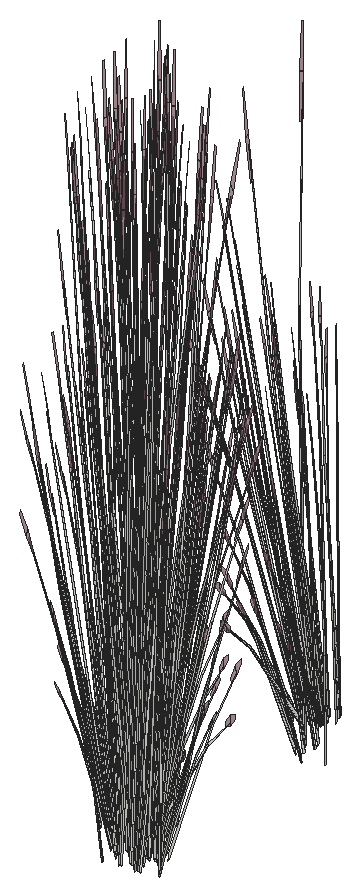
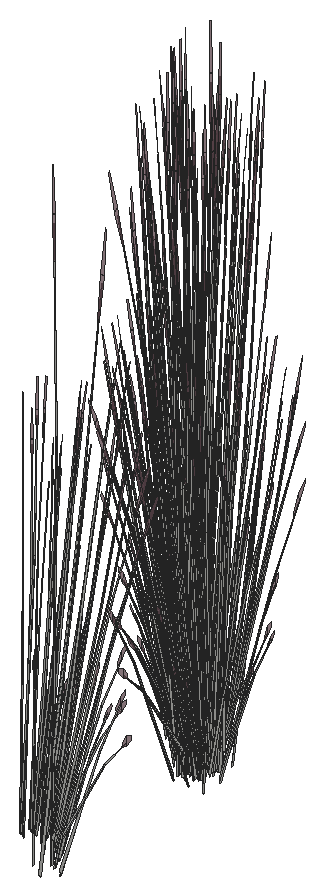
# SketchUp Ruby script. Lengths in inches.
U = 1.inch
M = Sketchup.active_model
def pt(a) = Geom::Point3d.new(a.map { |v| v * U })
def face(e, loops, mat)
  f = e.add_face(loops[0].map { |a| pt(a) })
  loops[1..].each { |l| e.add_face(l.map { |a| pt(a) }).erase! }
  f.material = f.back_material = mat if mat
  f
end
# faces: each face lists its corners as indices into pts; further lists are holes
def faces(e, pts, list, mat = nil) = list.each { |f| face(e, (f[0].is_a?(Array) ? f : [f]).map { |l| l.map { |i| pts[i] } }, mat) }
# xy, xz, yz: faces in a plane at the given z, y or x. An outline is a flat list of corners, or four numbers for a rectangle; further outlines are holes
def ring(l) = l.size == 4 ? [[l[0], l[1]], [l[2], l[1]], [l[2], l[3]], [l[0], l[3]]] : l.each_slice(2).to_a
def flat(e, list, mat, &to3) = list.each { |f| face(e, (f[0].is_a?(Array) ? f : [f]).map { |l| ring(l).map { |u, v| to3.(u, v) } }, mat) }
def xy(e, z, list, mat = nil) = flat(e, list, mat) { |x, y| [x, y, z] }
def xz(e, y, list, mat = nil) = flat(e, list, mat) { |x, z| [x, y, z] }
def yz(e, x, list, mat = nil) = flat(e, list, mat) { |y, z| [x, y, z] }
def lines(e, pts, list) = list.each { |a, b| e.add_line(pt(pts[a]), pt(pts[b])) }
# prism: a flat outline (further loops are holes) pulled along v
def prism(e, loops, v, mat = nil)
  f = face(e, loops, mat); d = Geom::Vector3d.new(v.map { |x| x * U })
  f.pushpull(f.normal.samedirection?(d) ? d.length : -d.length)
end
def box(e, o, s, mat = nil) = prism(e, [[o, [o[0] + s[0], o[1], o[2]], [o[0] + s[0], o[1] + s[1], o[2]], [o[0], o[1] + s[1], o[2]]]], [0, 0, s[2]], mat)
def at(x, y, z, deg = 0) = Geom::Transformation.translation(pt([x, y, z])) * Geom::Transformation.rotation(ORIGIN, Z_AXIS, deg.degrees)
def axes(o, x, y, z) = Geom::Transformation.new([*x, 0, *y, 0, *z, 0, *pt(o).to_a, 1])
def part(name) = M.definitions.add(name)
# library, detail: a bought-in or finely detailed component or shape, given as its bounding box
def library(name, o, s) = part(name).tap { |d| box(d.entities, o, s) }
def detail(e, o, s) = box(e.add_group.entities, o, s)
def put(e, d, t, mat = nil) = e.add_instance(d, t).tap { |i| i.material = mat if mat }
def group(e, t, mat = nil) = e.add_group.tap { |g| g.transformation = t; g.material = mat if mat }.entities
root = M.entities
M.materials.add("LightPink_Translucent").color = [144, 107, 117]
M.materials["LightPink_Translucent"].alpha = 0.75
c1 = part("blade")
p = [[2.15,0.21,22],[0,0.17,0],[0.09,0.45,0],[2.18,0.31,22],[2.29,0.31,22],[0.38,0.45,0],
  [2.48,0.24,33],[2.49,0.24,33],[2.48,0.22,33]]
faces(c1.entities,p,[[0,1,2,3],[4,5,2,3],[6,3,4,7],[8,0,3,6]])
c2 = part("seeds")
p = [[0.3,-0.1,1.38],[-0.01,-0.03,1.59],[-0.01,-0.03,0.03],[0.14,-0.07,-0.07],[0.29,-0.03,3],[0.15,0.01,3.11]]
faces(c2.entities,p,[[0,1,2,3],[1,0,4,5]],"LightPink_Translucent")
c3 = part("blade with seeds")
put(c3.entities,c1,at(0,0,0))
put(c3.entities,c2,axes([2.4,0.25,30.99],[1.5799,-0.05474,1.17369],[-0.12525,1.92788,0.29478],[-0.07173,-0.02425,1.56792]))
put(root,c3,axes([332.67,539,1402.53],[0.30722,-0.06665,-0.35414],[0.08112,0.381,0.4572],[0.08804,-0.10234,0.87481]))
put(root,c3,axes([329.78,538.36,1402.73],[0.01777,-0.35463,0.0643],[0.26836,0.00972,0.50621],[-0.1028,-0.03711,0.77189]))
put(root,c3,axes([330.71,539.55,1400.21],[0.17124,-0.42022,-0.44739],[0.35581,0.20224,0.21531],[0,-0.09687,1.43643]))
put(root,c3,axes([329.68,538.47,1402.53],[-0.20082,-0.29199,-0.35414],[0.2293,-0.2764,0.4572],[-0.1165,-0.04206,0.87481]))
put(root,c3,axes([330.86,539.34,1400.67],[-0.04113,-0.53214,-0.29095],[0.42835,-0.03218,-0.50002],[0.07543,-0.07088,1.59708]))
put(root,c3,axes([329.8,539.37,1400.03],[0.24637,-0.29097,-0.30978],[0.24637,0.29097,0.30978],[0,-0.09372,1.38974]))
put(root,c3,axes([329.7,537.97,1400.13],[-0.10181,0.3808,-0.03893],[-0.31336,-0.11714,-0.17649],[-0.04758,-0.06228,0.58215]))
put(root,c3,axes([332.42,539.22,1403.05],[-0.30722,0.06665,0.35414],[-0.08112,-0.381,-0.4572],[0.08804,-0.10234,0.87481]))
put(root,c3,axes([330.67,539.9,1400.67],[-0.39748,-0.22252,-0.29095],[0.19139,-0.46966,-0.50002],[-0.01249,-0.11531,1.59708]))
put(root,c3,axes([329.53,539.71,1400.375],[-0.44133,0,0],[0,-0.52122,-0.51607],[0,-0.11871,1.63711]))
put(root,c3,axes([329.61,538.78,1400.59],[0.06891,0.12984,1.43002],[-0.15879,0.35293,-0.30754],[-0.16304,-0.08436,0.61141]))
put(root,c3,axes([330.81,538.16,1400.03],[0.32928,0.11539,-0.30978],[-0.08291,0.40636,0.30978],[0.06638,-0.04686,1.38974]))
put(root,c3,axes([329.89,538.67,1402.98],[-0.35281,-0.01123,-0.71045],[0.0237,-0.47284,0.08574],[-0.14947,-0.0499,1.00501]))
put(root,c3,axes([332.7,539.16,1402.73],[0.2423,0.19613,0.0643],[-0.14107,0.2793,0.50621],[0.07768,-0.0903,0.77189]))
put(root,c3,axes([332.63,539.08,1402.73],[0.08753,0.42921,0.48003],[-0.34336,0.07449,0.3958],[0.1012,-0.10094,0.9933]))
put(root,c3,axes([333.55,539.6,1402.72],[0.04898,-0.07104,1.74944],[-0.06269,-0.43574,-0.27667],[0.12289,-0.08262,0.14031]))
put(root,c3,axes([329.875,539.58,1400.33],[-0.32829,0.39208,0.30756],[-0.32849,-0.38796,-0.36492],[-0.01146,-0.11134,1.64885]))
put(root,c3,axes([329.42,537.9,1402.71],[0.02617,0.04654,1.77383],[-0.12614,0.41836,-0.16761],[-0.12775,0.00303,0.31391]))
put(root,c3,axes([330.92,539.76,1400.43],[0.39767,0.22603,0.24065],[-0.19139,0.46966,0.50002],[0,-0.10827,1.60543]))
put(root,c3,axes([330.77,540.39,1400.4375],[0.09355,-0.55261,-0.23429],[0.44354,0.09633,0.51271],[-0.0775,-0.07631,1.5644]))
put(root,c3,axes([329.78,538.76,1402.68],[-0.25628,0.30892,-0.51099],[-0.22444,-0.32634,-0.3958],[-0.13021,-0.047,0.97773]))
put(root,c3,axes([329.97,538.625,1403.05],[0.20082,0.29199,0.35414],[-0.2293,0.2764,-0.4572],[-0.1165,-0.04206,0.87481]))
put(root,c3,axes([329.2,539.17,1400.77],[0.22533,-0.03337,1.1486],[-0.14293,0.29403,0.84392],[-0.11135,-0.04411,0.25299]))
put(root,c3,axes([330.79,539.44,1400.72],[-0.38326,0.02879,0.44739],[-0.03466,-0.47788,-0.21531],[0.06861,-0.04843,1.43643]))
put(root,c3,axes([329.91,538.4375,1403.03],[-0.0189,0.47427,-0.1216],[-0.35781,-0.01296,-0.67495],[-0.13781,-0.03295,1.02557]))
put(root,c3,axes([329.8,539.79,1400.48],[0,0.46636,0.49651],[-0.39487,0,0],[0,-0.10622,1.57504]))
put(root,c3,axes([332.59,540.26,1403.03],[-0.17758,-0.42229,-0.1216],[0.31518,-0.20752,-0.67495],[0.13282,-0.05572,1.02557]))
put(root,c3,axes([332.57,539.9,1402.68],[0.09562,-0.42421,-0.51099],[0.32782,0.1454,-0.3958],[0.13199,-0.0389,0.97773]))
put(root,c3,axes([332.06,538.17,1400.375],[0.22066,-0.46731,0],[0.36918,0.26061,-0.51607],[0.08408,0.05936,1.63711]))
put(root,c3,axes([329.46,539.09,1401.875],[0.14639,-0.01056,1.71376],[-0.09712,0.45778,0.13857],[-0.20862,-0.02831,0.73262]))
put(root,c3,axes([330.73,540.17,1400.21],[-0.21202,-0.39143,-0.44739],[0.32115,-0.27564,0.21531],[-0.06861,-0.04843,1.43643]))
put(root,c3,axes([330.78,539.62,1400.36],[0.15345,0.52148,0.45755],[-0.43845,0.18134,0.17955],[0.00536,-0.09582,1.58856]))
put(root,c3,axes([332.92,540.02,1399.98],[-0.22732,0.05597,1.41583],[-0.03618,-0.44548,0.08104],[0.15921,-0.06743,0.80566]))
put(root,c3,axes([333.34,539.62,1400.26],[-0.21881,-0.29821,-0.06488],[0.23965,-0.27324,-0.29416],[0.0679,-0.01924,0.97024]))
put(root,c3,axes([330.7,540.03,1400.72],[-0.17124,0.42022,0.44739],[-0.35581,-0.20224,-0.21531],[0,-0.09687,1.43643]))
put(root,c3,axes([331.33,539.66,1400.21],[0,-0.53961,0],[0.44133,0,0],[0,0,1.79456]))
put(root,c3,axes([331.87,538.41,1400.48],[-0.33032,-0.23318,0.49651],[0.19744,-0.41812,0],[0.07523,0.05311,1.57504]))
put(root,c3,axes([332.51,540.05,1402.98],[0.31014,-0.20596,-0.71045],[0.17284,0.42397,0.08574],[0.14985,-0.04816,1.00501]))
put(root,c3,axes([330.54,540.32,1400.06],[-0.36714,-0.07646,-0.62353],[0.07747,-0.47163,-0.16365],[-0.10956,-0.05715,1.37633]))
put(root,c3,axes([331.12,539.32,1400.36],[-0.29264,0.42323,0.45755],[-0.34767,-0.3736,0.17955],[0.07055,-0.04224,1.58856]))
put(root,c3,axes([331.44,540.08,1400.3],[-0.32829,-0.4014,-0.06131],[0.32849,-0.40164,0],[-0.01146,-0.01402,1.75571]))
put(root,c3,axes([330.61,538.625,1400.47],[-0.10196,0.46348,0.17642],[-0.3731,-0.13116,0.35086],[0.06445,-0.00226,1.60407]))
put(root,c3,axes([332.47,540.13,1403.05],[-0.29332,-0.1301,0.35414],[0.08555,-0.37955,-0.4572],[0.11809,-0.0348,0.87481]))
put(root,c3,axes([329.4,539.4375,1402.73],[0.09971,-0.42522,0.48003],[0.32782,0.1454,0.3958],[-0.12892,0.02555,0.9933]))
put(root,c3,axes([330.46,539,1399.59],[-0.3474,0.18671,1.28929],[-0.11057,-0.53572,0.50096],[0.21332,0.00891,1.46642]))
put(root,c3,axes([331.39,539.14,1400.62],[0.06809,-0.4162,0.1448],[0.33266,0.07225,-0.41347],[0.06054,0.04274,1.26744]))
put(root,c3,axes([329.37,539.33,1402.73],[-0.12963,-0.31798,0.0643],[0.23638,-0.15564,0.50621],[-0.1042,0.03071,0.77189]))
put(root,c3,axes([330.82,540.13,1400.36],[0.44609,0.09826,0.45755],[-0.09078,0.55493,0.17955],[-0.06519,-0.05359,1.58856]))
put(root,c3,axes([333.17,539.72,1399.49],[-0.01845,-0.0708,1.76342],[0.12793,-0.41416,-0.26939],[0.12905,-0.00596,0.30037]))
put(root,c3,axes([329.36,539.65,1399.49],[0.00895,0.0735,1.76342],[-0.18044,0.38382,-0.26939],[-0.12817,-0.01935,0.30037]))
put(root,c3,axes([331.25,539.25,1400.72],[-0.21202,-0.39143,0.44739],[0.32115,-0.27564,-0.21531],[0.06861,0.04843,1.43643]))
put(root,c3,axes([330.15,541.04,1400.03],[-0.08291,-0.40636,-0.30978],[0.32928,-0.11539,0.30978],[-0.06638,-0.04686,1.38974]))
put(root,c3,axes([330.58,541.01,1400.47],[0.37926,-0.12378,0.17642],[0.09365,0.46065,0.35086],[-0.03382,-0.06712,1.60407]))
put(root,c3,axes([331.36,539.27,1400.67],[0.35635,-0.30962,-0.29095],[0.23697,0.43749,-0.50002],[0.08792,0.04443,1.59708]))
put(root,c3,axes([332.78,540.09,1402.53],[0.29332,0.1301,-0.35414],[-0.08555,0.37955,0.4572],[0.11809,-0.0348,0.87481]))
put(root,c3,axes([330.0625,541.21,1400.02],[-0.33032,-0.23318,-0.49651],[0.19744,-0.41812,0],[-0.07523,-0.05311,1.57504]))
put(root,c3,axes([332.26,538.45,1400.02],[0.33032,0.23318,-0.49651],[-0.19744,0.41812,0],[0.07523,0.05311,1.57504]))
put(root,c3,axes([329.33,539.49,1402.53],[-0.29332,-0.1301,-0.35414],[0.08555,-0.37955,0.4572],[-0.11809,0.0348,0.87481]))
put(root,c3,axes([331.63,539.78,1400.21],[0.39487,0,0],[0,0.48281,0],[0,0,1.78407]))
put(root,c3,axes([330.96,540.39,1400.67],[-0.35635,0.30962,-0.29095],[-0.23697,-0.43749,-0.50002],[-0.08792,-0.04443,1.59708]))
put(root,c3,axes([331.74,538.65,1400.47],[-0.37926,0.12378,0.17642],[-0.09365,-0.46065,0.35086],[0.03382,0.06712,1.60407]))
put(root,c3,axes([331.98,539.62,1401.875],[-0.14639,0.01056,1.71376],[0.09712,-0.45778,0.13857],[0.20862,0.02831,0.73262]))
put(root,c3,axes([332.17,538.625,1400.03],[0.08291,0.40636,-0.30978],[-0.32928,0.11539,0.30978],[0.06638,0.04686,1.38974]))
put(root,c3,axes([332.73,540.25,1402.73],[0.12963,0.31798,0.0643],[-0.23638,0.15564,0.50621],[0.1042,-0.03071,0.77189]))
put(root,c3,axes([331.5,539.53,1400.38],[-0.44609,-0.09826,0.49198],[0.09078,-0.55493,0.19306],[0.06519,0.05359,1.70813]))
put(root,c3,axes([332.71,540.14,1402.73],[-0.09971,0.42522,0.48003],[-0.32782,-0.1454,0.3958],[0.12892,-0.02555,0.9933]))
put(root,c3,axes([331.15,540.9,1400.2],[-0.11516,-0.40207,0],[0.32884,-0.1408,0],[0,0,1.54371]))
put(root,c3,axes([330.93,540.52,1400.62],[-0.06809,0.4162,0.1448],[-0.33266,-0.07225,-0.41347],[-0.06054,-0.04274,1.26744]))
put(root,c3,axes([329.64,539.44,1403.05],[0.29332,0.1301,0.35414],[-0.08555,0.37955,-0.4572],[-0.11809,0.0348,0.87481]))
put(root,c3,axes([331.58,540.85,1400.18],[0.37054,-0.15823,-0.19198],[0.1302,0.45581,0.00008],[0.0409,-0.01749,1.73897]))
put(root,c3,axes([331.71,541.04,1400.47],[0.10196,-0.46348,0.17642],[0.3731,0.13116,0.35086],[-0.06445,0.00226,1.60407]))
put(root,c3,axes([331.62,539.99,1400.21],[0.24637,0.30123,0],[-0.24637,0.30123,0],[0,0,1.69266]))
put(root,c3,axes([330.22,539.42,1401.34],[0.10032,-0.06746,1.77064],[0.0346,0.47103,0.13857],[-0.2173,0.0625,0.63284]))
put(root,c3,axes([332.29,539.86,1400.47],[-0.2773,-0.3397,0.17642],[0.27945,-0.32949,0.35086],[-0.03063,0.06937,1.60407]))
put(root,c3,axes([331.78,539.34,1400.06],[0.36714,0.07646,-0.62353],[-0.07747,0.47163,-0.16365],[0.10956,0.05715,1.37633]))
put(root,c3,axes([333.4,540.17,1400.77],[-0.21807,0.07699,1.1486],[0.10265,-0.31819,0.84392],[0.11568,0.02177,0.25299]))
put(root,c3,axes([331.07,541.09,1400.2],[-0.35581,-0.20937,0],[0.17124,-0.43505,0],[0,0,1.62707]))
put(root,c3,axes([331.36,540.53,1400.46],[-0.34464,-0.37536,-0.25192],[0.29,-0.42149,0.5513],[-0.0928,0.04391,1.68216]))
put(root,c3,axes([330.45,541.25,1400.48],[0.33032,0.23318,0.49651],[-0.19744,0.41812,0],[-0.07523,-0.05311,1.57504]))
put(root,c3,axes([331.62,539.64,1400.72],[0.17124,-0.42022,0.44739],[0.35581,0.20224,-0.21531],[0,0.09687,1.43643]))
put(root,c3,axes([333.3,541.51,1402.71],[-0.03191,-0.04083,1.77383],[0.06981,-0.43764,-0.16761],[0.12571,-0.02796,0.31391]))
put(root,c3,axes([329.14,539.74,1402.72],[-0.05763,0.06055,1.74944],[0.0049,0.44239,-0.27667],[-0.13211,0.05753,0.14031]))
put(root,c3,axes([331.55,539.875,1400.29],[0,0.53934,-0.05637],[-0.44133,0,0],[0,0.01695,1.79368]))
put(root,c3,axes([329.53,539.68,1402.68],[-0.09562,0.42421,-0.51099],[-0.32782,-0.1454,-0.3958],[-0.13199,0.0389,0.97773]))
put(root,c3,axes([329.51,539.32,1403.03],[0.17758,0.42229,-0.1216],[-0.31518,0.20752,-0.67495],[-0.13282,0.05572,1.02557]))
put(root,c3,axes([331.58,539.49,1400.21],[0.21202,0.39143,-0.44739],[-0.32115,0.27564,0.21531],[0.06861,0.04843,1.43643]))
put(root,c3,axes([333.02,541.15,1401.93],[-0.06755,-0.39203,-0.03492],[0.31928,-0.09013,-0.15832],[0.06667,0.02485,0.52218]))
put(root,c3,axes([330.26,541.49,1400.375],[-0.22066,0.46731,0],[-0.36918,-0.26061,-0.51607],[-0.08408,-0.05936,1.63711]))
put(root,c3,axes([332.19,541.14,1403.03],[0.0189,-0.47427,-0.1216],[0.35781,0.01296,-0.67495],[0.13781,0.03295,1.02557]))
put(root,c3,axes([332.52,539.87,1400.48],[0,-0.46636,0.49651],[0.39487,0,0],[0,0.10622,1.57504]))
put(root,c3,axes([331.53,540.22,1400.72],[0.38326,-0.02879,0.44739],[0.03466,0.47788,-0.21531],[-0.06861,0.04843,1.43643]))
put(root,c3,axes([331.77,539.73,1400.62],[0.32884,-0.136,0.1448],[0.11516,0.38837,-0.41347],[0,0.08547,1.26744]))
put(root,c3,axes([332.14,540.95,1403.05],[-0.20082,-0.29199,0.35414],[0.2293,-0.2764,-0.4572],[0.1165,0.04206,0.87481]))
put(root,c3,axes([331.1875,540.45,1400.21],[-0.38326,0.02879,-0.44739],[-0.03466,-0.47788,0.21531],[-0.06861,0.04843,1.43643]))
put(root,c3,axes([332.99,540.68,1400.59],[-0.085,-0.1147,1.43002],[0.1106,-0.37943,-0.30754],[0.17198,0.0514,0.61141]))
put(root,c3,axes([331.47,541.09,1400.2],[0.35581,0.20937,0],[-0.17124,0.43505,0],[0,0,1.74954]))
put(root,c3,axes([332.5,540.85,1402.72],[0.07571,-0.00789,1.74944],[0.20767,-0.36231,-0.27667],[0.13467,0.04783,0.14031]))
put(root,c3,axes([331.61,541.56,1400.19],[-0.21791,-0.46895,-0.05142],[0.36918,-0.26061,0.51607],[-0.09097,0.04465,1.6363]))
put(root,c3,axes([331.53,540.42,1400.62],[0.26075,0.2802,0.1448],[-0.2175,0.31612,-0.41347],[-0.06054,0.04274,1.26744]))
put(root,c3,axes([329.47,540.5,1402.73],[-0.08753,-0.42921,0.48003],[0.34336,-0.07449,0.3958],[-0.1012,0.10094,0.9933]))
put(root,c3,axes([329.41,540.41,1402.73],[-0.2423,-0.19613,0.0643],[0.14107,-0.2793,0.50621],[-0.07768,0.0903,0.77189]))
put(root,c3,axes([329.52,539.9,1401.875],[0.12246,-0.09864,1.71376],[0.1031,0.45582,0.13857],[-0.19225,0.10302,0.73262]))
put(root,c3,axes([332.21,540.91,1402.98],[0.35281,0.01123,-0.71045],[-0.0237,0.47284,0.08574],[0.14947,0.0499,1.00501]))
put(root,c3,axes([331.8125,541.29,1400.48],[0.33032,-0.23318,0.49651],[0.19744,0.41812,0],[-0.07523,0.05311,1.57504]))
put(root,c3,axes([331.34,540.92,1400.29],[0.15345,0.53576,-0.06012],[-0.43845,0.18773,0],[0.00536,0.01871,1.72173]))
put(root,c3,axes([331.51,541.5,1400.03],[-0.32928,-0.11539,-0.30978],[0.08291,-0.40636,0.30978],[-0.06638,0.04686,1.38974]))
put(root,c3,axes([329.14,540.67,1400.59],[0.12266,0.03828,1.43002],[0.07906,0.39104,-0.30754],[-0.16661,0.0732,0.61141]))
put(root,c3,axes([329.6875,540.35,1403.05],[0.30722,-0.06665,0.35414],[0.08112,0.381,-0.4572],[-0.08804,0.10234,0.87481]))
put(root,c3,axes([332.78,539.95,1400.375],[0.44133,0,0],[0,0.52122,-0.51607],[0,0.11871,1.63711]))
put(root,c3,axes([328.5,540.18,1402.71],[0.04504,0.01251,1.77383],[0.13934,0.41205,-0.16761],[-0.0922,0.10815,0.31391]))
put(root,c3,axes([332.61,540.22,1400.2],[-0.44111,-0.00373,-0.04976],[0,-0.52122,0.49943],[-0.01386,0.11865,1.58352]))
put(root,c3,axes([331.65,539.76,1400.67],[0.39748,0.22252,-0.29095],[-0.19139,0.46966,-0.50002],[0.01249,0.11531,1.59708]))
put(root,c3,axes([328.88,541.49,1400.77],[0.14709,-0.21136,1.1486],[0.05804,0.3346,0.84392],[-0.1063,0.05991,0.25299]))
put(root,c3,axes([332.42,541.1,1402.53],[0.20082,0.29199,-0.35414],[-0.2293,0.2764,0.4572],[0.1165,0.04206,0.87481]))
put(root,c3,axes([332.52,540.29,1400.03],[-0.24637,0.29097,-0.30978],[-0.24637,-0.29097,0.30978],[0,0.09372,1.38974]))
put(root,c3,axes([331.46,540.32,1400.67],[0.04113,0.53214,-0.29095],[-0.42835,0.03218,-0.50002],[-0.07543,0.07088,1.59708]))
put(root,c3,axes([332.32,541.22,1402.73],[-0.01777,0.35463,0.0643],[-0.26836,-0.00972,0.50621],[0.1028,0.03711,0.77189]))
put(root,c3,axes([331.61,540.11,1400.21],[-0.17124,0.42022,-0.44739],[-0.35581,-0.20224,0.21531],[0,0.09687,1.43643]))
put(root,c3,axes([329.43,540.58,1402.53],[-0.30722,0.06665,-0.35414],[-0.08112,-0.381,0.4572],[-0.08804,0.10234,0.87481]))
put(root,c3,axes([332.34,541.1,1402.73],[-0.26024,0.30729,0.48003],[-0.22444,-0.32634,0.3958],[0.1221,0.05668,0.9933]))
put(root,c3,axes([328.99,541.4375,1403.65],[0.31145,0.12449,-0.06488],[-0.0958,0.38314,-0.29416],[-0.05094,0.05817,0.97024]))
put(root,c3,axes([331.2,540.73,1400.06],[-0.23773,0.35053,-0.62353],[-0.29532,-0.31785,-0.16365],[-0.09526,0.08744,1.37633]))
put(root,c3,axes([331.52,541.46,1403.05],[-0.05451,-0.37564,0.35414],[0.31161,-0.09919,-0.4572],[0.0837,0.10765,0.87481]))
put(root,c3,axes([331.62,541.32,1400.33],[0.44186,0.15158,0.30756],[-0.11054,0.54181,-0.36492],[-0.07313,0.06781,1.64885]))
put(root,c3,axes([331.59,541.68,1400.02],[-0.33032,0.23318,-0.49651],[-0.19744,-0.41812,0],[-0.07523,0.05311,1.57504]))
put(root,c3,axes([332.6875,540.3,1400.02],[0,0.46636,-0.49651],[-0.39487,0,0],[0,0.10622,1.57504]))
put(root,c3,axes([331.7,540.35,1401.875],[-0.1311,-0.08035,1.71376],[0.27131,-0.33708,0.13857],[0.16909,0.15206,0.73262]))
put(root,c3,axes([331.72,539.3,1402.47],[-0.30498,-0.24231,1.38283],[0.32203,-0.37727,0.59665],[0.0984,0.22736,1.33663]))
put(root,c3,axes([329.53,540.32,1403.03],[0.32648,0.25715,-0.1216],[-0.18809,0.3724,-0.67495],[-0.09224,0.12945,1.02557]))
put(root,c3,axes([332.18,541.27,1400.77],[-0.19872,-0.13409,1.1486],[0.2566,-0.13625,0.84392],[0.06921,0.11541,0.25299]))
put(root,c3,axes([331.49,541.65,1403.03],[0.21031,-0.39918,-0.1216],[0.30457,0.22997,-0.67495],[0.10587,0.11278,1.02557]))
put(root,c3,axes([329.97,540.2,1401.875],[0.08815,-0.14329,1.71376],[0.22258,0.38678,0.13857],[-0.15267,0.17614,0.73262]))
put(root,c3,axes([329.6875,540.625,1402.68],[0.09067,0.42583,-0.51099],[-0.34336,0.07449,-0.3958],[-0.0984,0.11438,0.97773]))
put(root,c3,axes([330.1,541.11,1403.05],[0.23881,-0.24554,0.35414],[0.22606,0.28036,-0.4572],[-0.0344,0.14245,0.87481]))
put(root,c3,axes([331.89,541.61,1400.375],[0.22066,0.46731,0],[-0.36918,0.26061,-0.51607],[-0.08408,0.05936,1.63711]))
put(root,c3,axes([331.21,541.98,1402.71],[0.00104,-0.05646,1.77383],[0.30246,-0.2491,-0.16761],[0.10506,0.08891,0.31391]))
put(root,c3,axes([332.24,541.77,1399.49],[0.02571,-0.06733,1.76342],[0.32373,-0.19829,-0.26939],[0.09815,0.10263,0.30037]))
put(root,c3,axes([331.7,539.76,1400.84],[-0.00964,-0.43909,1.41272],[0.43635,0.11382,0.59816],[-0.1032,0.24027,1.3335]))
put(root,c3,axes([331.8125,540.24,1400.09],[0.12941,0.42699,-0.69212],[-0.37279,0.15378,-0.18165],[0.0143,0.14459,1.52773]))
put(root,c3,axes([329.88,541.34,1402.73],[-0.29004,-0.02173,0.0643],[0.00795,-0.32812,0.50621],[-0.03035,0.12569,0.77189]))
put(root,c3,axes([329.27,541.71,1399.49],[0.04734,0.04659,1.76342],[0.08027,0.4317,-0.26939],[-0.10492,0.09206,0.30037]))
put(root,c3,axes([329.98,541.37,1402.73],[-0.25132,-0.3182,0.48003],[0.2669,-0.27442,0.3958],[-0.04636,0.14929,0.9933]))
put(root,c3,axes([331.74,541.45,1402.68],[0.34827,-0.11086,-0.51099],[0.06092,0.41983,-0.3958],[0.09354,0.12031,0.97773]))
put(root,c3,axes([330.77,541.52,1403.05],[0.1064,-0.35863,0.35414],[0.31043,0.1046,-0.4572],[0.02846,0.14439,0.87481]))
put(root,c3,axes([332.22,541.88,1400.67],[-0.22633,-0.01463,1.0506],[0.14947,-0.31064,0.58006],[0.08941,0.11036,0.8241]))
put(root,c3,axes([331.56,541.8,1402.73],[-0.16041,0.29625,0.0643],[-0.22843,-0.17248,0.50621],[0.07385,0.09498,0.77189]))
put(root,c3,axes([331.1875,542.8,1403.65],[0.2439,-0.26754,-0.06488],[0.22348,0.29302,-0.29416],[0.01573,0.08303,0.97024]))
put(root,c3,axes([331.63,541.72,1402.73],[-0.35104,0.10702,0.48003],[-0.06092,-0.41983,0.3958],[0.08256,0.12373,0.9933]))
put(root,c3,axes([329.9,540.56,1401.875],[0.06572,-0.16029,1.71376],[0.27569,0.33172,0.13857],[-0.12437,0.20675,0.73262]))
put(root,c3,axes([331.48,541.125,1400.59],[0.00623,-0.15459,1.43002],[0.29764,-0.17268,-0.30754],[0.09188,0.18503,0.61141]))
put(root,c3,axes([330.67,541.84,1402.73],[-0.26007,0.1585,0.0643],[-0.12729,-0.28902,0.50621],[0.02512,0.1274,0.77189]))
put(root,c3,axes([329.98,541.46,1402.53],[-0.23881,0.24554,-0.35414],[-0.22606,-0.28036,0.4572],[-0.0344,0.14245,0.87481]))
put(root,c3,axes([329.15,541.39,1402.72],[-0.00877,0.09229,1.74944],[0.24897,0.32105,-0.27667],[-0.06518,0.15182,0.14031]))
put(root,c3,axes([329.95,541.18,1403.4],[0.3879,0.02311,-0.13498],[-0.0106,0.43749,-0.74919],[-0.02694,0.1685,1.13838]))
put(root,c3,axes([330.67,541.67,1403.03],[0.34538,-0.21713,-0.1216],[0.16972,0.38536,-0.67495],[0.04557,0.16239,1.02557]))
put(root,c3,axes([330.77,541.8125,1403.0625],[-0.34777,-0.12192,0.53283],[0.11892,-0.40083,0.43934],[0.0209,0.15763,1.10256]))
put(root,c3,axes([330.13,542.42,1400.77],[-0.00913,-0.2773,1.1486],[0.22824,0.19778,0.84392],[-0.04489,0.13217,0.25299]))
put(root,c3,axes([330.73,541.75,1399.49],[0.05712,-0.02538,1.76342],[0.34359,0.13968,-0.26939],[0.01005,0.15742,0.30037]))
put(root,c3,axes([330.21,541.35,1403],[0.25266,0.31335,-0.5672],[-0.2669,0.27442,-0.43934],[-0.03844,0.15921,1.08528]))
put(root,c3,axes([329.9375,541.82,1400.82],[0.32063,-0.08258,0.06507],[0.07371,0.33271,-0.86304],[-0.02033,0.16842,0.7736]))
put(root,c3,axes([330.96,541.65,1402.68],[0.34695,0.11691,-0.51099],[-0.11892,0.40083,-0.3958],[0.03181,0.16138,0.97773]))
put(root,c3,axes([331.16,540.82,1401.875],[-0.08068,-0.14973,1.71376],[0.3728,-0.12606,0.13857],[0.08426,0.23506,0.73262]))
put(root,c3,axes([330.8,541.9,1402.53],[-0.1064,0.35863,-0.35414],[-0.31043,-0.1046,0.4572],[0.02846,0.14439,0.87481]))
put(root,c3,axes([330.13,541.2,1403.34],[-0.00918,0.43138,-0.7886],[-0.38672,-0.02897,0.09517],[-0.04081,0.18275,1.11556]))
put(root,c3,axes([329.125,542.34,1402.71],[0.04004,-0.02816,1.77383],[0.33095,0.18728,-0.16761],[-0.00778,0.15594,0.31391]))
put(root,c3,axes([330.5,540.9,1401.875],[-0.00864,-0.17899,1.71376],[0.37441,0.11874,0.13857],[-0.02316,0.25508,0.73262]))
put(root,c3,axes([330.84,541.57,1402.98],[0.16845,0.3792,-0.71045],[-0.34676,0.21133,0.08574],[0.03939,0.18322,1.00501]))
put(root,c3,axes([329.86,542.17,1400.59],[0.11138,-0.07357,1.43002],[0.27499,0.22183,-0.30754],[-0.08185,0.19194,0.61141]))
put(root,c3,axes([330.58,542.53,1402.72],[0.04474,0.0751,1.74944],[0.36104,0.0295,-0.27667],[0.03631,0.16562,0.14031]))
put(root,c3,axes([330.01,541.81,1401.36],[0.00775,-0.24075,1.54345],[0.34877,0.12716,0.21329],[-0.03022,0.25658,0.72882]))
put(root,c3,axes([330.27,558.84,1401.875],[0.08068,0.14973,1.71376],[-0.3728,0.12606,0.13857],[-0.08426,-0.23506,0.73262]))
put(root,c3,axes([330.89,557.85,1402.72],[-0.05398,-0.06539,1.74944],[-0.36026,0.04145,-0.27667],[-0.0575,-0.15639,0.14031]))
put(root,c3,axes([331.72,558.62,1400.59],[-0.10032,0.0944,1.43002],[-0.30046,-0.16522,-0.30754],[0.05569,-0.20547,0.61141]))
put(root,c3,axes([331.27,558.95,1402.98],[-0.16845,-0.3792,-0.71045],[0.34676,-0.21133,0.08574],[-0.03939,-0.18322,1.00501]))
put(root,c3,axes([330.17,558.44,1400.59],[-0.02137,0.15256,1.43002],[-0.31245,0.12771,-0.30754],[-0.07303,-0.19719,0.61141]))
put(root,c3,axes([330.98,558.11,1399.49],[-0.0592,0.0168,1.76342],[-0.32738,-0.18913,-0.26939],[0.00549,-0.15776,0.30037]))
put(root,c3,axes([331.97,559.32,1402.98],[0.00918,-0.43138,-0.71045],[0.38672,0.02897,0.08574],[0.04081,-0.18275,1.00501]))
put(root,c3,axes([332.51,558.65,1402.72],[-0.00341,-0.09282,1.74944],[-0.28775,-0.26825,-0.27667],[0.04449,-0.16261,0.14031]))
put(root,c3,axes([331.3,558.63,1402.53],[0.1064,-0.35863,-0.35414],[0.31043,0.1046,0.4572],[-0.02846,-0.14439,0.87481]))
put(root,c3,axes([331.53,559.1,1401.875],[-0.06572,0.16029,1.71376],[-0.27569,-0.33172,0.13857],[0.12437,-0.20675,0.73262]))
put(root,c3,axes([332.43,558.31,1402.71],[-0.03584,0.03562,1.77383],[-0.35118,-0.12018,-0.16761],[-0.01271,-0.15545,0.31391]))
put(root,c3,axes([331.14,558.875,1402.68],[-0.34695,-0.11691,-0.51099],[0.11892,-0.40083,-0.3958],[-0.03181,-0.16138,0.97773]))
put(root,c3,axes([331.35,557.87,1400.77],[0.04528,0.27194,1.1486],[-0.25117,-0.15062,0.84392],[0.02703,-0.13924,0.25299]))
put(root,c3,axes([331.89,559.18,1402.68],[-0.25266,-0.31335,-0.51099],[0.2669,-0.27442,-0.3958],[0.03844,-0.15921,0.97773]))
put(root,c3,axes([330.52,557.63,1402.71],[-0.00658,0.0559,1.77383],[-0.32474,0.20287,-0.16761],[-0.09556,-0.1037,0.31391]))
put(root,c3,axes([330.45,558.625,1403.09],[0.39316,-0.11987,0.53763],[0.06823,0.47021,0.4433],[-0.09247,-0.13858,1.11249]))
put(root,c3,axes([331.34,558.71,1402.73],[0.34777,0.12192,0.48003],[-0.11892,0.40083,0.3958],[-0.0209,-0.15763,0.9933]))
put(root,c3,axes([331.4375,558.86,1403.03],[-0.34538,0.21713,-0.1216],[-0.16972,-0.38536,-0.67495],[-0.04557,-0.16239,1.02557]))
put(root,c3,axes([332.15,559.34,1403.03],[-0.3879,-0.02311,-0.1216],[0.0106,-0.43749,-0.67495],[0.02694,-0.1685,1.02557]))
put(root,c3,axes([332.13,559.0625,1402.53],[0.23881,-0.24554,-0.35414],[0.22606,0.28036,0.4572],[0.0344,-0.14245,0.87481]))
put(root,c3,axes([330.0625,558.2,1400.77],[0.18411,0.16231,1.1486],[-0.26813,0.09757,0.84392],[-0.05737,-0.12474,0.25299]))
put(root,c3,axes([331.43,558.68,1402.73],[0.26007,-0.1585,0.0643],[0.12729,0.28902,0.50621],[-0.02512,-0.1274,0.77189]))
put(root,c3,axes([330.51,559.06,1402.98],[-0.30095,-0.22541,-0.71045],[0.21388,-0.395,0.08574],[-0.10904,-0.13459,1.00501]))
put(root,c3,axes([330.4,558.76,1402.53],[-0.05451,-0.37564,-0.35414],[0.31161,-0.09919,0.4572],[-0.0837,-0.10765,0.87481]))
put(root,c3,axes([330.54,558.73,1402.73],[0.16041,-0.29625,0.0643],[0.22843,0.17248,0.50621],[-0.07385,-0.09498,0.77189]))
put(root,c3,axes([329.92,558.6875,1399.49],[-0.03419,0.06144,1.76342],[-0.3455,0.13246,-0.26939],[-0.08346,-0.12049,0.30037]))
put(root,c3,axes([330.49,560.375,1400.1],[-0.14494,-0.47823,-0.69835],[0.41752,-0.17223,-0.18329],[-0.01602,-0.16194,1.54149]))
put(root,c3,axes([329.73,559.31,1401.875],[0.1311,0.08035,1.71376],[-0.27131,0.33708,0.13857],[-0.16909,-0.15206,0.73262]))
put(root,c3,axes([332.43,558.91,1399.49],[-0.05283,-0.03674,1.76342],[-0.13569,-0.41045,-0.26939],[0.09154,-0.11138,0.30037]))
put(root,c3,axes([331.33,559.01,1403.05],[-0.1064,0.35863,0.35414],[-0.31043,-0.1046,-0.4572],[-0.02846,-0.14439,0.87481]))
put(root,c3,axes([330.37,559.07,1402.68],[-0.34827,0.11086,-0.51099],[-0.06092,-0.41983,-0.3958],[-0.09354,-0.12031,0.97773]))
put(root,c3,axes([332.125,559.16,1402.73],[0.25132,0.3182,0.48003],[-0.2669,0.27442,0.3958],[0.04636,-0.14929,0.9933]))
put(root,c3,axes([330.61,558.7,1403.43],[-0.23555,0.44708,-0.13619],[-0.34112,-0.25757,-0.75594],[-0.11858,-0.12631,1.14864]))
put(root,c3,axes([332.22,559.1875,1402.73],[0.29004,0.02173,0.0643],[-0.00795,0.32812,0.50621],[0.03035,-0.12569,0.77189]))
put(root,c3,axes([332,559.41,1403.05],[-0.23881,0.24554,0.35414],[-0.22606,-0.28036,-0.4572],[0.0344,-0.14245,0.87481]))
put(root,c3,axes([332.42,560.07,1402.98],[0.18436,-0.36797,-0.71045],[0.32306,0.26151,0.08574],[0.11008,-0.13332,1.00501]))
put(root,c3,axes([330.43,559,1400.375],[-0.22066,-0.46731,0],[0.36918,-0.26061,-0.51607],[0.08408,-0.05936,1.63711]))
put(root,c3,axes([332.41,559.9,1402.68],[-0.09067,-0.42583,-0.51099],[0.34336,-0.07449,-0.3958],[0.0984,-0.11438,0.97773]))
put(root,c3,axes([330.92,558.4375,1400.13],[-0.2439,0.26754,-0.03893],[-0.22348,-0.29302,-0.17649],[-0.01573,-0.08303,0.58215]))
put(root,c3,axes([329.71,558.57,1402.72],[-0.07594,-0.00329,1.74944],[-0.24177,0.32918,-0.27667],[-0.129,-0.06726,0.14031]))
put(root,c3,axes([332.58,560.2,1403.03],[-0.32648,-0.25715,-0.1216],[0.18809,-0.3724,-0.67495],[0.09224,-0.12945,1.02557]))
